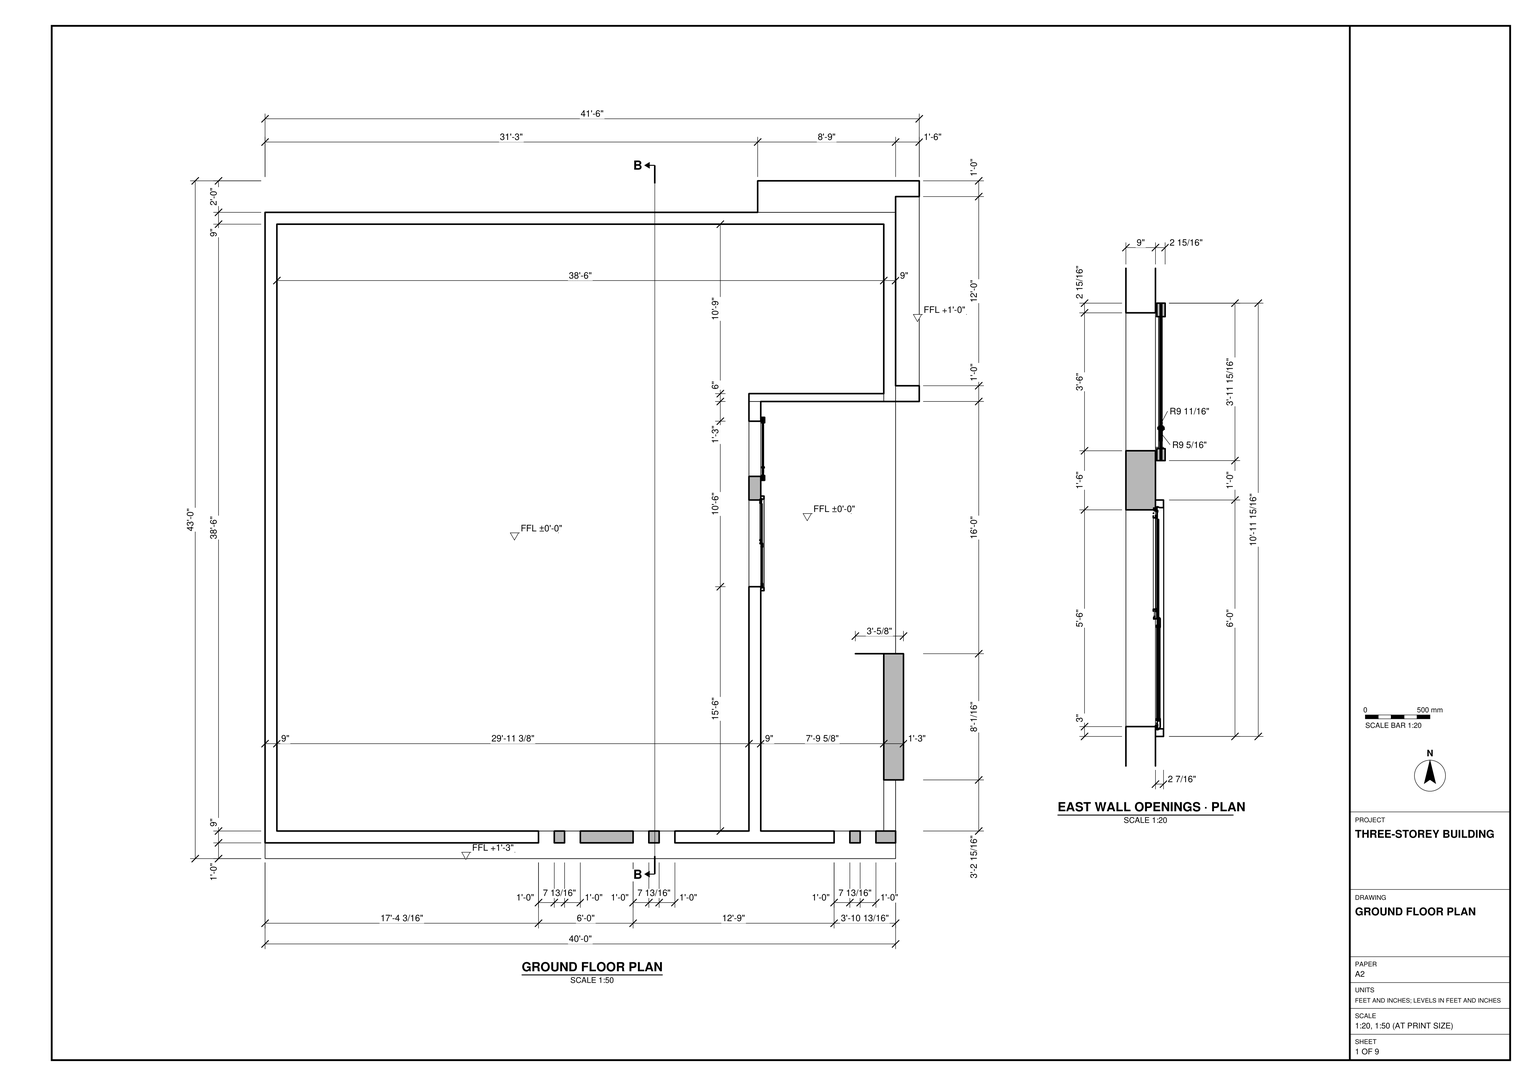
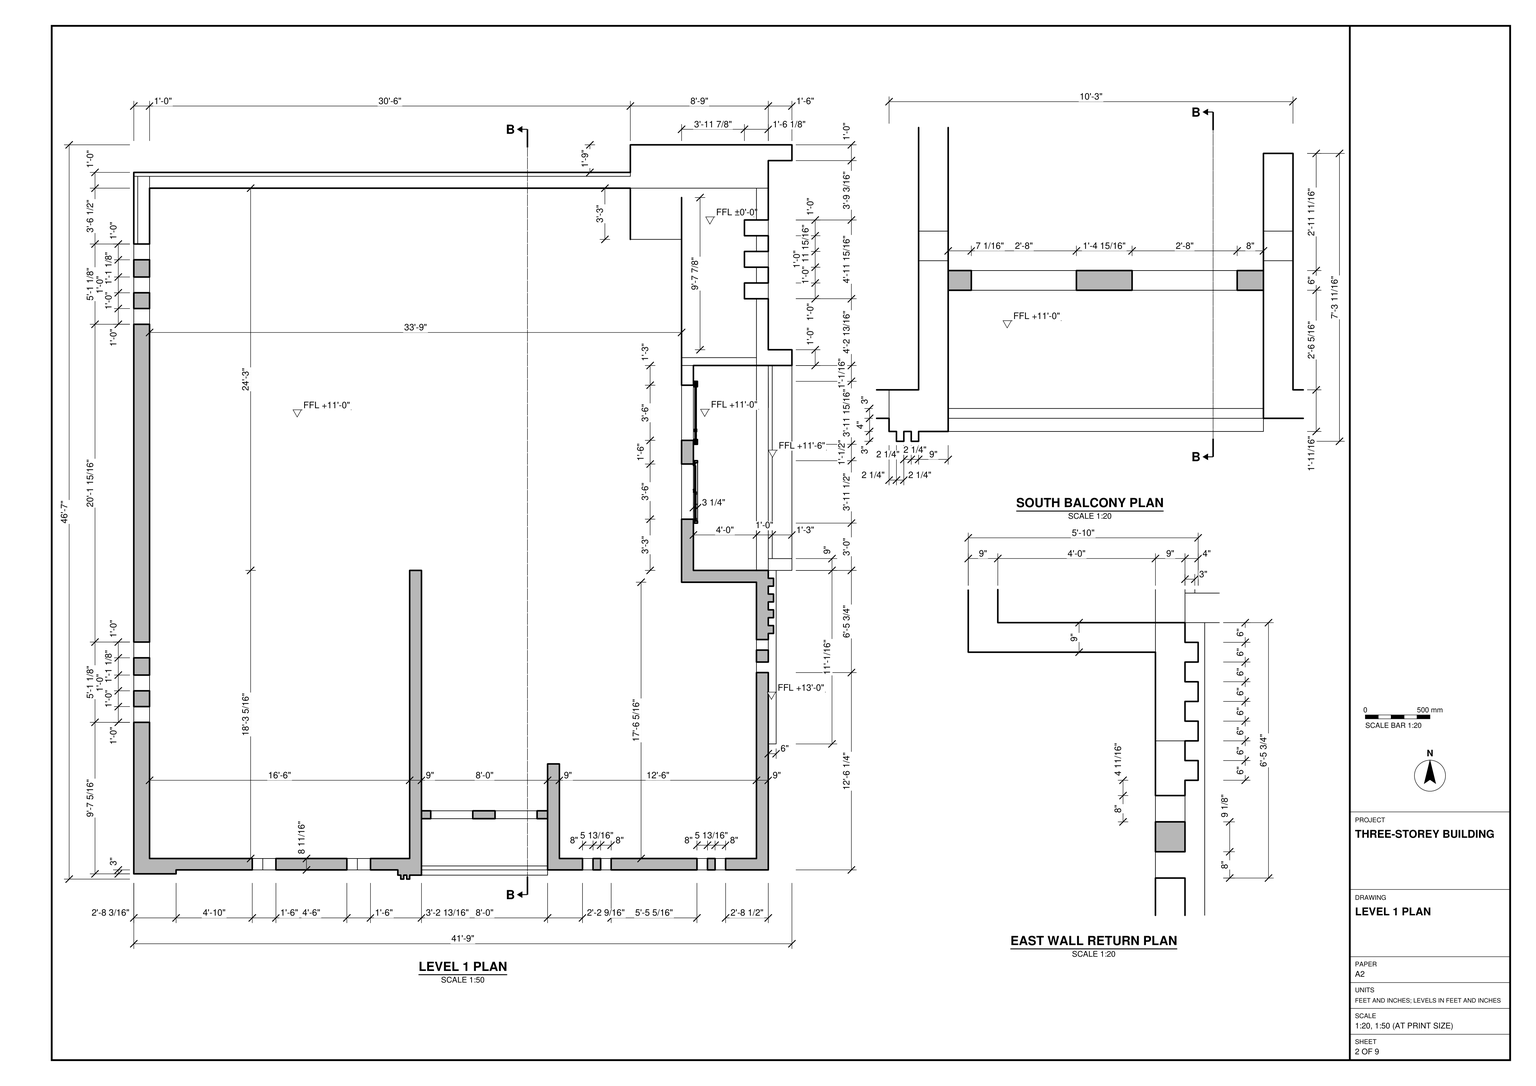
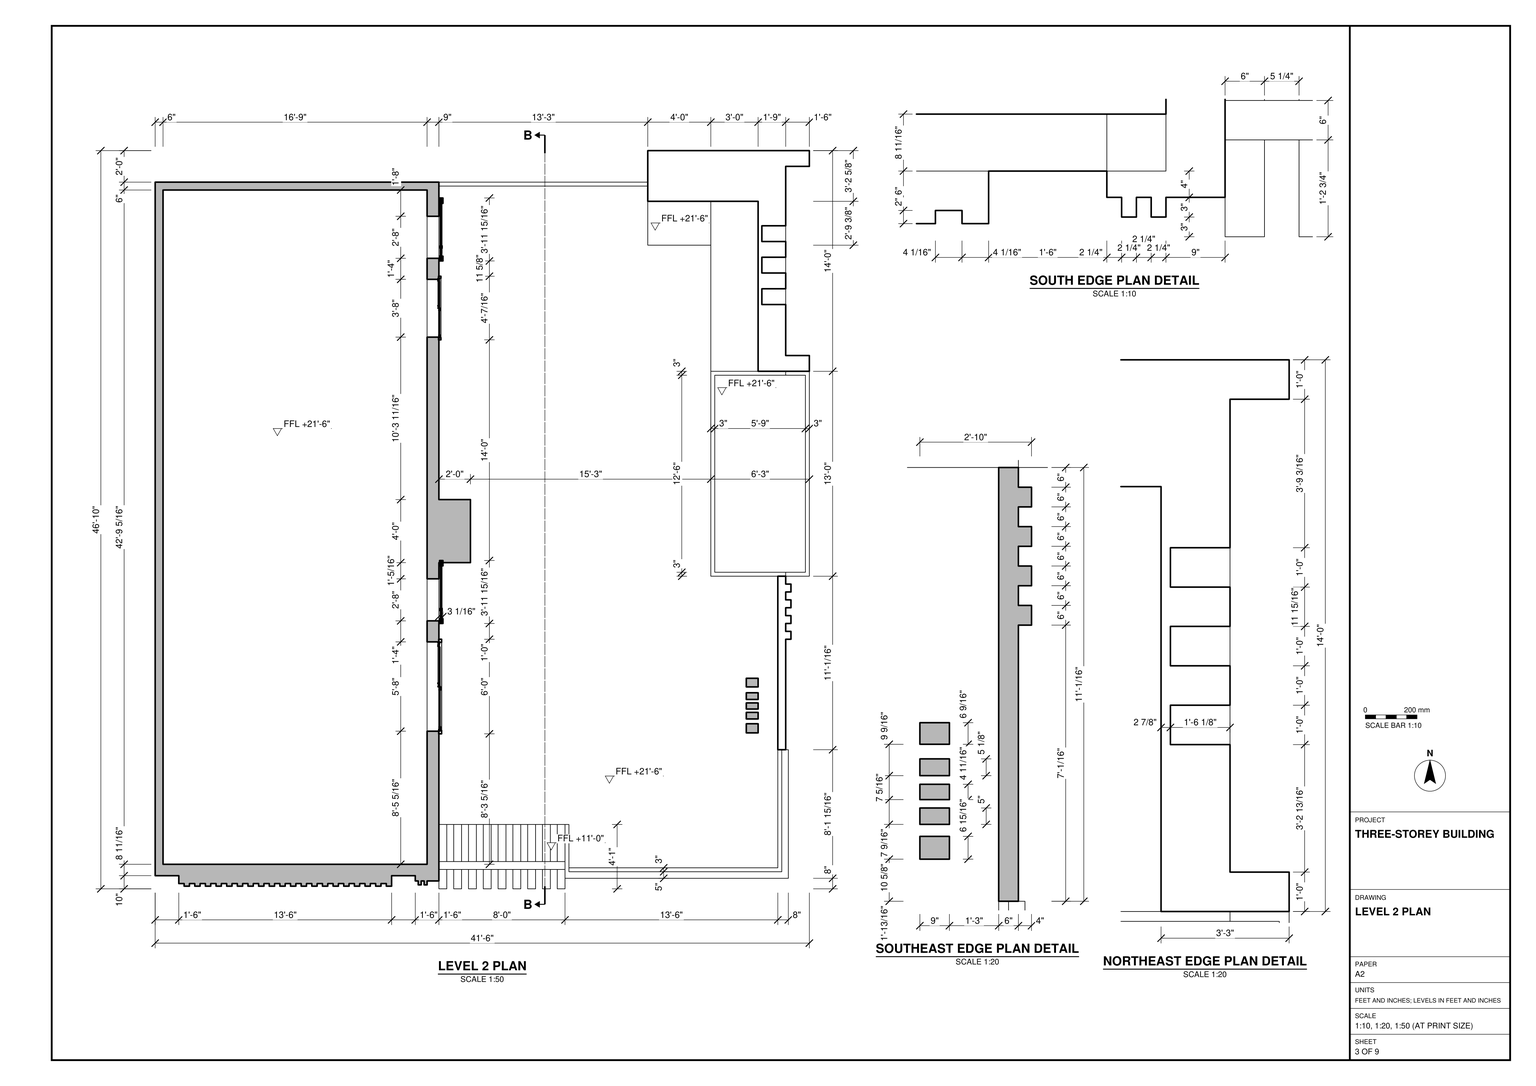
Build the three-storey building in SketchUp from task_files/diagram_01.pdf. Work in feet and inches. The overall model extents are 53'-5 5/16" along X, 49'-10 3/8" along Y and 37'-0" in height. Set the ground floor at ±0'-0", Level 1 at +11'-0" and Level 2 at +21'-6". Use the dimensioned wall lines on each plan, rather than the overall model extents, to lay out each floor.

On the ground floor, form the wide north end and the recessed east side. Use the east wall detail to place the openings and the pier between them. At Level 1, set the south balcony between the two projecting bays. Include the grouped west wall openings and the stepped return on the east side. At Level 2, distinguish the long enclosed space on the west from the open terrace on the east. Follow the enlarged details for the projections and recesses along the terrace edges.

Model the walls at their drawn thicknesses, with floor slabs, roof, door and window units, and balcony and terrace edges as shown. Include stairs, built-in joinery and main furniture where drawn. Keep shell elements such as walls, slabs and roof, and each furniture or joinery piece, in separate groups or components. Use components for repeated parts. Decor and loose items may be any suitable library components. Save one SketchUp model as output_files/three_storey_building_with_recessed_balcony_and_terrace.skp.

# SketchUp Ruby script. Lengths in inches.
U = 1.inch
M = Sketchup.active_model
def pt(a) = Geom::Point3d.new(a.map { |v| v * U })
def face(e, loops, mat)
  f = e.add_face(loops[0].map { |a| pt(a) })
  loops[1..].each { |l| e.add_face(l.map { |a| pt(a) }).erase! }
  f.material = f.back_material = mat if mat
  f
end
# faces: each face lists its corners as indices into pts; further lists are holes
def faces(e, pts, list, mat = nil) = list.each { |f| face(e, (f[0].is_a?(Array) ? f : [f]).map { |l| l.map { |i| pts[i] } }, mat) }
# xy, xz, yz: faces in a plane at the given z, y or x. An outline is a flat list of corners, or four numbers for a rectangle; further outlines are holes
def ring(l) = l.size == 4 ? [[l[0], l[1]], [l[2], l[1]], [l[2], l[3]], [l[0], l[3]]] : l.each_slice(2).to_a
def flat(e, list, mat, &to3) = list.each { |f| face(e, (f[0].is_a?(Array) ? f : [f]).map { |l| ring(l).map { |u, v| to3.(u, v) } }, mat) }
def xy(e, z, list, mat = nil) = flat(e, list, mat) { |x, y| [x, y, z] }
def xz(e, y, list, mat = nil) = flat(e, list, mat) { |x, z| [x, y, z] }
def yz(e, x, list, mat = nil) = flat(e, list, mat) { |y, z| [x, y, z] }
def lines(e, pts, list) = list.each { |a, b| e.add_line(pt(pts[a]), pt(pts[b])) }
# prism: a flat outline (further loops are holes) pulled along v
def prism(e, loops, v, mat = nil)
  f = face(e, loops, mat); d = Geom::Vector3d.new(v.map { |x| x * U })
  f.pushpull(f.normal.samedirection?(d) ? d.length : -d.length)
end
def box(e, o, s, mat = nil) = prism(e, [[o, [o[0] + s[0], o[1], o[2]], [o[0] + s[0], o[1] + s[1], o[2]], [o[0], o[1] + s[1], o[2]]]], [0, 0, s[2]], mat)
def at(x, y, z, deg = 0) = Geom::Transformation.translation(pt([x, y, z])) * Geom::Transformation.rotation(ORIGIN, Z_AXIS, deg.degrees)
def axes(o, x, y, z) = Geom::Transformation.new([*x, 0, *y, 0, *z, 0, *pt(o).to_a, 1])
def part(name) = M.definitions.add(name)
# library, detail: a bought-in or finely detailed component or shape, given as its bounding box
def library(name, o, s) = part(name).tap { |d| box(d.entities, o, s) }
def detail(e, o, s) = box(e.add_group.entities, o, s)
def put(e, d, t, mat = nil) = e.add_instance(d, t).tap { |i| i.material = mat if mat }
def group(e, t, mat = nil) = e.add_group.tap { |g| g.transformation = t; g.material = mat if mat }.entities
root = M.entities
M.materials.add("Brick_20_1K").color = [186, 180, 162]
M.materials.add("D01_Frost_White").color = [255, 242, 206]
M.materials.add("Glass_Basic_01").color = [161, 173, 186]
M.materials["Glass_Basic_01"].alpha = 0.25
M.materials.add("M05_Graphite_Haze").color = [114, 114, 114]
M.materials.add("M08_Obsidian_Black").color = [30, 30, 30]
M.materials.add("ThomThom - Waistcoat1").color = [155, 155, 155]
M.materials.add("Wood_Veneer_15_1K").color = [153, 101, 54]
M.materials.add("[Color_009]1").color = [0, 0, 0]
c1 = library("2016+Honda+Civic+LX+Sedan",[0.01,0.03,0.02],[16.17,34.46,10.62])
c2 = library("porta+4",[0.2,-5.42,1.33],[46.55,4.72,83.21])
c3 = library("mesh-165",[-1596.32,-2661.67,-39.91],[1702.88,1739.15,82.5])
c4 = part("Group15")
put(c4.entities,c3,at(294.66,859.51,3.5))
xy(root,288,[[240,556,399,559]])
xz(root,556,[[240,258,399,288]],"Glass_Basic_01")
xz(root,559,[[240,258,399,288]],"Glass_Basic_01")
p = [[504,451,96.6875],[504,571,96.6875]]
lines(root,p,[[0,1]])
put(root,c1,axes([537.55,376.82,0.04],[6.42482,0,0],[0,6.42482,0],[0,0,6.42482]))
g1 = group(root,at(33,88,0))
box(g1,[-9,-9,-6],[480,480,6])
g2 = group(root,at(24,79,0))
xy(g2,0,[[0,-12,0,480,375,480,375,504,498,504,498,336,471,336,471,471,9,471,9,9,368.36,9,368.36,336,377.36,336,377.36,9,471,9,471,144,486,144,486,47.91,480,47.91,480,-12],[368.36,336,471,342]])
xy(g2,7.84,[[368.36,279,377.36,321]])
xy(g2,12,[[480,348,498,492]],"M05_Graphite_Haze")
xy(g2,15,[[0,-12,480,-12,480,0,465.02,0,465.02,9,453.02,9,453.02,0,445.1875,0,445.1875,9,433.1875,9,433.1875,0,312,0,312,9,300,9,300,0,292.16,0,292.16,9,280.16,9,280.16,0,240,0,240,9,228,9,228,0,220.16,0,220.16,9,208.16,9,208.16,0,0,0],[471,9,480,47.91]])
xy(g2,43.84,[[368.36,195,377.36,261]])
xy(g2,51,[[68.23,0,76.23,9],[152.16,0,160.16,9]],"[Color_009]1")
xy(g2,75,[[423,336,453,342]],"Wood_Veneer_15_1K")
xy(g2,97.84,[[368.36,195,377.36,261],[368.36,279,377.36,321]])
xy(g2,99,[[68.23,0,76.23,9],[152.16,0,160.16,9]],"M05_Graphite_Haze")
xy(g2,105,[[423,336,453,342]],"Wood_Veneer_15_1K")
xy(g2,111,[[433.1875,0,445.1875,9],[453.02,0,465.02,9],[471,9,480,47.91]],"M05_Graphite_Haze")
xy(g2,111,[[208.16,0,220.16,9],[228,0,240,9],[280.16,0,292.16,9],[300,0,312,9]],"[Color_009]1")
xy(g2,114,[[200.25,-55,200.25,-52,198,-52,198,0,312,0,312,-52,207,-52,207,-55,204.75,-55,204.75,-52,202.5,-52,202.5,-55]],"[Color_009]1")
xy(g2,120,[[0,-48,198,0],[312,-48,480,0],[0,0,480,0,480,9,377.36,9,377.36,336,368.36,336,368.36,9,0,9],[0,9,9,480],[9,9,9,471,471,471,471,342,368.36,342,368.36,9],
  [368.36,336,471,342]])
xy(g2,120,[[471,144,486,180]],"Brick_20_1K")
xy(g2,120,[[377.36,9,377.36,336,498,336,498,180,471,180,471,9]],"Wood_Veneer_15_1K")
xy(g2,132,[[216,-45,312,-9],[9,-39.33,207,-39.33,207,180,216,180,216,-3,312,-3,312,32.67,321,32.67,321,-39.33,471,-39.33,471,171,414,171,414,432,375,432,375,471,9,471],[216,-9,312,-3],[423,180,471,336],[471,180,480,336],
  [480,180,480.43,180,480,336]])
xy(g2,134,[[272,-9,304,-3]])
xy(g2,135,[[414,279,423,321]])
xy(g2,138,[[480,189,480.4,189,480,336],[480.4,189,483,189,483,336,480,336],[483,189,498,336]])
xy(g2,139.39,[[-3,-51,0,480],[0,-51,29.1875,-48],[-3,480,375,483]],"Wood_Veneer_15_1K")
xy(g2,144,[[216,-52,312,-48],[216,-48,312,-45]])
xy(g2,145.98,[[338.59,-48,346.59,-39.33],[352.39,-48,360.39,-39.33],[425.71,-48,433.71,-39.33],[439.51,-48,447.51,-39.33]],"M08_Obsidian_Black")
xy(g2,150.99,[[-3,64.33,9,76.33],[-3,88.33,9,100.33],[-3,113.46,9,125.46],[-3,367.37,9,379.37],[-3,391.37,9,403.37],
  [-3,416.49,9,428.49]],"Wood_Veneer_15_1K")
xy(g2,156,[[480,47.91,486,47.91,486,180,480,180,480,174,484,174,484,168,480,168,480,162,484,162,484,156,480,156,480,150,484,150,484,144,480,144,480,138,484,138,484,132,480,132,480,110.23,471,110.23,471,102.23,480,102.23],[471,119.34,480,127.34]])
xy(g2,161.03,[[461.85,386.83,480,398.83],[461.85,410.83,480,422.83],[461.85,434.79,480,446.79]],"M05_Graphite_Haze")
xy(g2,168,[[480,180,498,189],[480,189,483,336]])
xy(g2,168,[[87.19,-48,95.19,-39.33],[95.19,-48,105.19,-39.33],[159.19,-48,167.19,-39.33],[167.19,-48,177.19,-39.33],[216,-48,312,-45]],"M08_Obsidian_Black")
xy(g2,170,[[223.05,-9,255.05,-3]])
xy(g2,171,[[414,219,423,261]])
xy(g2,202,[[223.05,-9,255.05,-3]])
xy(g2,213,[[414,219,423,261],[414,279,423,321]])
xy(g2,214,[[272,-9,304,-3]])
xy(g2,217.98,[[338.59,-48,346.59,-39.33],[352.39,-48,360.39,-39.33],[425.71,-48,433.71,-39.33],[439.51,-48,447.51,-39.33],[471,102.23,480,110.23],
  [471,119.34,480,127.34]],"M08_Obsidian_Black")
xy(g2,222.99,[[-3,64.33,9,76.33],[-3,88.33,9,100.33],[-3,113.46,9,125.46],[-3,367.37,9,379.37],[-3,391.37,9,403.37],
  [-3,416.49,9,428.49]],"Wood_Veneer_15_1K")
xy(g2,233.03,[[461.85,386.83,480,398.83],[461.85,410.83,480,422.83],[461.85,434.79,480,446.79]],"M05_Graphite_Haze")
xy(g2,240,[[87.19,-48,105.19,-39.33],[159.19,-48,177.19,-39.33]],"M08_Obsidian_Black")
xy(g2,240,[[-3,-51,29.1875,-51,29.1875,-48,0,-48,0,480,375,480,375,483,-3,483]],"Wood_Veneer_15_1K")
xy(g2,252,[[198,-48,198,-39.33,9,-39.33,9,471,312,471,312,-3,216,-3,216,180,207,180,207,-48],[321,-39.33,321,471,375,471,375,432,414,432,414,171,471,171,471,-39.33],[312,32.67,321,471],[414,171,471,171,471,180,423,180,423,432,414,432],[423,180,498,336]])
xy(g2,252,[[216,-52,222,-9],[227.26,-52,233.26,-9],[238.53,-52,244.53,-9],[249.79,-52,255.79,-9],[261.05,-52,267.05,-9],
  [272.3125,-52,278.3125,-9],[283.58,-52,289.58,-9],[294.84,-52,300.84,-9],[306.1,-52,312,-9]],"Wood_Veneer_15_1K")
xy(g2,258,[[198,-48,207,-39.33],[222,-43.25,227.26,-37.25],[227.26,-43.25,233.26,-37.25],[233.26,-43.25,238.53,-37.25],[238.53,-43.25,244.53,-37.25],
  [244.53,-43.25,249.79,-37.25],[249.79,-43.25,255.79,-37.25],[255.79,-43.25,261.05,-37.25],[261.05,-43.25,267.05,-37.25],[267.05,-43.25,272.3125,-37.25],
  [272.3125,-43.25,278.3125,-37.25],[278.3125,-43.25,283.58,-37.25],[283.58,-43.25,289.58,-37.25],[289.58,-43.25,294.84,-37.25],[294.84,-43.25,300.84,-37.25],
  [300.84,-43.25,306.1,-37.25],[306.1,-43.25,312,-37.25],[[315,-42,474,-42,474,180,423,180,423,432,375,432,375,480,216,480,216,238.34,240,238.34,240,190.34,216,190.34,216,-9,315,-9],[450,60.73,459,67.67],[450,95.72,459,102.29],[450,86.16,459,91.27],[450,71.32,459,76.32],[450,78.87,459,83.53]],[6,-39.33,207,474],[207,180,216,180,216,190.34,240,190.34,240,238.34,216,238.34,216,474,207,474],
  [423,180,480,180,480,183,426,183,426,333,480,333,480,336,423,336],[426,183,495,333],[423,336,459,465.39],[375,432,423,465.39]])
xy(g2,258,[[216,-58,222,-43.25],[227.26,-58,233.26,-43.25],[238.53,-58,244.53,-43.25],[249.79,-58,255.79,-43.25],[261.05,-58,267.05,-43.25],
  [272.3125,-58,278.3125,-43.25],[283.58,-58,289.58,-43.25],[294.84,-58,300.84,-43.25],[306.1,-58,312,-43.25],[216,-37.25,222,-9],
  [227.26,-37.25,233.26,-9],[238.53,-37.25,244.53,-9],[249.79,-37.25,255.79,-9],[261.05,-37.25,267.05,-9],[272.3125,-37.25,278.3125,-9],
  [283.58,-37.25,289.58,-9],[294.84,-37.25,300.84,-9],[306.1,-37.25,312,-9]],"Wood_Veneer_15_1K")
xy(g2,260,[[207,146,216,178],[207,422,216,454]])
xy(g2,264,[[216,-43.25,312,-37.25]],"Wood_Veneer_15_1K")
xy(g2,270,[[312,-48,480,-48,480,47.91,477,47.91,477,-45,315,-45,315,-9,312,-9],[315,-45,477,-45,477,47.91,474,47.91,474,-42,315,-42],[480,180,498,180,498,336,480,336,480,333,495,333,495,183,480,183]])
xy(g2,276,[[22.05,-56,22.05,-54,18,-54,18,-48,180,-48,180,-56,175.95,-56,175.95,-54,171.9,-54,171.9,-56,167.85,-56,167.85,-54,163.8,-54,163.8,-56,159.75,-56,159.75,-54,155.7,-54,155.7,-56,151.65,-56,151.65,-54,147.6,-54,147.6,-56,143.55,-56,143.55,-54,139.5,-54,139.5,-56,135.45,-56,135.45,-54,131.4,-54,131.4,-56,127.35,-56,127.35,-54,123.3,-54,123.3,-56,119.25,-56,119.25,-54,115.2,-54,115.2,-56,111.15,-56,111.15,-54,107.1,-54,107.1,-56,103.05,-56,103.05,-54,99,-54,99,-56,94.95,-56,94.95,-54,90.9,-54,90.9,-56,86.85,-56,86.85,-54,82.8,-54,82.8,-56,78.75,-56,78.75,-54,74.7,-54,74.7,-56,70.65,-56,70.65,-54,66.6,-54,66.6,-56,62.55,-56,62.55,-54,58.5,-54,58.5,-56,54.45,-56,54.45,-54,50.4,-54,50.4,-56,46.35,-56,46.35,-54,42.3,-54,42.3,-56,38.25,-56,38.25,-54,34.2,-54,34.2,-56,30.15,-56,30.15,-54,26.1,-54,26.1,-56]],"ThomThom - Waistcoat1")
xy(g2,287,[[312,-50,480,-48],[480,-50,482,47.91]],"Glass_Basic_01")
xy(g2,288,[[312,-50,482,-50,482,47.91,477,47.91,477,-45,315,-45,315,-9,312,-9]])
xy(g2,288,[[480,180,498,180,498,336,480,336,480,333,495,333,495,183,480,183]],"Glass_Basic_01")
xy(g2,290.04,[[461.85,386.83,480,398.83],[461.85,410.83,480,422.83],[461.85,434.79,480,446.79]],"M05_Graphite_Haze")
xy(g2,296,[[207,62,216,130],[207,362,216,406]])
xy(g2,312,[[474,47.91,480,47.91,480,132,484,132,484,138,480,138,480,144,484,144,484,150,480,150,480,156,484,156,484,162,480,162,480,168,484,168,484,174,480,174,480,180,474,180]])
xy(g2,340,[[207,62,216,130],[207,146,216,178],[207,362,216,406],[207,422,216,454]])
xy(g2,362.04,[[461.85,386.83,480,398.83],[461.85,410.83,480,422.83],[461.85,434.79,480,446.79]],"M05_Graphite_Haze")
xy(g2,366,[[22.05,-56,26.1,-56,26.1,-54,30.15,-54,30.15,-56,34.2,-56,34.2,-54,38.25,-54,38.25,-56,42.3,-56,42.3,-54,46.35,-54,46.35,-56,50.4,-56,50.4,-54,54.45,-54,54.45,-56,58.5,-56,58.5,-54,62.55,-54,62.55,-56,66.6,-56,66.6,-54,70.65,-54,70.65,-56,74.7,-56,74.7,-54,78.75,-54,78.75,-56,82.8,-56,82.8,-54,86.85,-54,86.85,-56,90.9,-56,90.9,-54,94.95,-54,94.95,-56,99,-56,99,-54,103.05,-54,103.05,-56,107.1,-56,107.1,-54,111.15,-54,111.15,-56,115.2,-56,115.2,-54,119.25,-54,119.25,-56,123.3,-56,123.3,-54,127.35,-54,127.35,-56,131.4,-56,131.4,-54,135.45,-54,135.45,-56,139.5,-56,139.5,-54,143.55,-54,143.55,-56,147.6,-56,147.6,-54,151.65,-54,151.65,-56,155.7,-56,155.7,-54,159.75,-54,159.75,-56,163.8,-56,163.8,-54,167.85,-54,167.85,-56,171.9,-56,171.9,-54,175.95,-54,175.95,-56,180,-56,180,-48,18,-48,18,-54,22.05,-54]],"ThomThom - Waistcoat1")
xy(g2,372,[[216,190.34,240,238.34]])
xy(g2,384,[[[-24,-79,312,504],[-18,-73,306,498]],[[-18,-73,306,498],[200.25,-55,202.5,-55,202.5,-52,204.75,-52,204.75,-55,207,-55,207,-52,216,-52,216,480,0,480,0,-48,198,-48,198,-52,200.25,-52]],[200.25,-55,200.25,-52,198,-52,198,-48,0,-48,0,-39.33,216,-39.33,216,-52,207,-52,207,-55,204.75,-55,204.75,-52,202.5,-52,202.5,-55],[0,-39.33,6,480],[6,-39.33,207,474],
  [207,-39.33,216,474],[6,474,216,480]])
xy(g2,390,[[-18,-73,306,498]])
xy(g2,390.94,[[312,5.5,312,26.83,417.58,26.83,417.58,48.15,312,48.15,312,102.29,417.35,102.29,417.35,112.125,312,112.125,312,133.45,417.58,133.45,417.58,154.78,312,154.78,312,176.1,417.58,176.1,417.58,197.43,312,197.43,312,218.75,417.35,218.75,417.35,240.08,312,240.08,312,261.4,417.35,261.4,417.35,282.73,312,282.73,312,304.05,417.35,304.05,417.35,325.375,312,325.375,312,346.7,417.35,346.7,417.35,368.03,312,368.03,312,389.35,417.35,389.35,417.35,410.68,312,410.68,312,432,450,432,450,5.5]])
xy(g2,409.59,[[312,5.5,366,26.83],[366,5.5,450,5.5,450,60.73,366,60.73,366,48.15,417.58,48.15,417.58,26.83,366,26.83],[312,48.15,366,60.73],[366,60.73,450,67.67],[312,67.67,366,69.48],
  [366,67.67,450,69.48],[312,69.48,366,71.32],[366,69.48,450,71.32],[366,71.32,450,76.32],[312,76.32,366,78.87],
  [366,76.32,450,78.87],[366,78.87,450,83.53],[312,83.53,366,86.16],[366,83.53,450,86.16],[366,86.16,450,90.8],
  [366,90.8,450,91.27],[312,91.27,366,95.72],[366,91.27,450,95.72],[366,95.72,450,102.29],[417.35,102.29,450,102.29,450,432,312,432,312,410.68,417.35,410.68,417.35,389.35,312,389.35,312,368.03,417.35,368.03,417.35,346.7,312,346.7,312,325.375,417.35,325.375,417.35,304.05,312,304.05,312,282.73,417.35,282.73,417.35,261.4,312,261.4,312,240.08,417.35,240.08,417.35,218.75,312,218.75,312,197.43,417.58,197.43,417.58,176.1,312,176.1,312,154.78,417.58,154.78,417.58,133.45,312,133.45,312,112.125,417.35,112.125]])
xy(g2,415.59,[[312,60.73,459,67.67],[312,71.32,459,76.32],[312,78.87,459,83.53],[312,86.16,459,91.27],[312,95.72,459,102.29]])
xy(g2,426,[[-24,-79,312,-79,312,465.39,306,465.39,306,-73,-18,-73,-18,465.39,-24,465.39],[-24,465.39,-18,504],[-18,465.39,306,498],[306,465.39,312,504],[312,465.39,375,504],
  [-18,498,306,504]])
xy(g2,426,[[480,348,498,492]],"M05_Graphite_Haze")
xy(g2,438,[[459,336,498,336,498,504,-24,504,-24,465.39,459,465.39]])
xz(g2,-79,[[-24,384,312,426]])
xz(g2,-73,[[-18,390,306,426]])
xz(g2,-58,[[216,255,222,258],[227.26,255,233.26,258],[238.53,255,244.53,258],[249.79,255,255.79,258],[261.05,255,267.05,258],
  [272.3125,255,278.3125,258],[283.58,255,289.58,258],[294.84,255,300.84,258],[306.1,255,312,258]],"Wood_Veneer_15_1K")
xz(g2,-56,[[22.05,276,26.1,366],[30.15,276,34.2,366],[38.25,276,42.3,366],[46.35,276,50.4,366],[54.45,276,58.5,366],
  [62.55,276,66.6,366],[70.65,276,74.7,366],[78.75,276,82.8,366],[86.85,276,90.9,366],[94.95,276,99,366],
  [103.05,276,107.1,366],[111.15,276,115.2,366],[119.25,276,123.3,366],[127.35,276,131.4,366],[135.45,276,139.5,366],
  [143.55,276,147.6,366],[151.65,276,155.7,366],[159.75,276,163.8,366],[167.85,276,171.9,366],[175.95,276,180,366]],"ThomThom - Waistcoat1")
xz(g2,-55,[[200.25,114,202.5,384],[204.75,114,207,384]])
xz(g2,-54,[[18,276,22.05,366],[26.1,276,30.15,366],[34.2,276,38.25,366],[42.3,276,46.35,366],[50.4,276,54.45,366],
  [58.5,276,62.55,366],[66.6,276,70.65,366],[74.7,276,78.75,366],[82.8,276,86.85,366],[90.9,276,94.95,366],
  [99,276,103.05,366],[107.1,276,111.15,366],[115.2,276,119.25,366],[123.3,276,127.35,366],[131.4,276,135.45,366],
  [139.5,276,143.55,366],[147.6,276,151.65,366],[155.7,276,159.75,366],[163.8,276,167.85,366],[171.9,276,175.95,366]],"ThomThom - Waistcoat1")
xz(g2,-52,[[198,114,200.25,384],[202.5,114,204.75,384]])
xz(g2,-52,[[207,114,312,114,312,144,216,144,216,384,207,384]],"M05_Graphite_Haze")
xz(g2,-51,[[-3,139.39,29.1875,240]],"Wood_Veneer_15_1K")
xz(g2,-50,[[312,287,482,288]],"M08_Obsidian_Black")
xz(g2,-48,[[[0,120,198,120,198,384,0,384,0,240,29.1875,240,29.1875,139.39,0,139.39],[18,276,180,366],[159.19,168,177.19,240],[87.19,168,105.19,240]],[312,120,480,132],[312,246,480,270],[198,252,207,258]])
xz(g2,-48,[[216,144,312,168],[312,270,480,287]],"Glass_Basic_01")
xz(g2,-48,[[[312,132,480,246],[439.51,145.98,447.51,217.98],[338.59,145.98,346.59,217.98],[352.39,145.98,360.39,217.98],[425.71,145.98,433.71,217.98]]],"Wood_Veneer_15_1K")
xz(g2,-45,[[216,132,312,144],[216,144,312,168],[315,270,477,288]],"Glass_Basic_01")
xz(g2,-43.25,[[216,258,312,264]],"Wood_Veneer_15_1K")
xz(g2,-42,[[315,258,474,270]])
xz(g2,-39.33,[[[9,132,9,252,198,252,198,258,207,258,207,132],[87.19,168,105.19,240],[159.19,168,177.19,240]],[[321,132,471,252],[352.39,145.98,360.39,217.98],[338.59,145.98,346.59,217.98],[439.51,145.98,447.51,217.98],[425.71,145.98,433.71,217.98]],[6,258,207,384]])
xz(g2,-37.25,[[216,258,312,264]],"Wood_Veneer_15_1K")
xz(g2,-12,[[0,0,480,15]])
xz(g2,-9,[[[216,132,270,132,270,216,306,216,306,132,312,132,312,252,306.1,252,306.1,258,300.84,258,300.84,252,294.84,252,294.84,258,289.58,258,289.58,252,283.58,252,283.58,258,278.3125,258,278.3125,252,272.3125,252,272.3125,258,267.05,258,267.05,252,261.05,252,261.05,258,255.79,258,255.79,252,249.79,252,249.79,258,244.53,258,244.53,252,238.53,252,238.53,258,233.26,258,233.26,252,227.26,252,227.26,258,222,258,222,252,216,252],[221.05,168,257.05,204]],[[270,132,306,216],[272,134,304,214]],[[221.05,168,257.05,204],[223.05,170,255.05,202]],[227.26,252,233.26,258],[238.53,252,244.53,258],
  [249.79,252,255.79,258],[261.05,252,267.05,258],[272.3125,252,278.3125,258],[283.58,252,289.58,258],[294.84,252,300.84,258],
  [306.1,252,312,258],[312,252,312.1,258],[312,258,315,270],[312,270,315,288]])
xz(g2,-3,[[[216,132,312,252],[272,134,304,214],[223.05,170,255.05,202]]])
xz(g2,0,[[198,114,312,120]])
xz(g2,0,[[[0,15,208.16,15,208.16,111,220.16,111,220.16,15,228,15,228,111,240,111,240,15,280.16,15,280.16,111,292.16,111,292.16,15,300,15,300,111,312,111,312,114,198,114,198,120,0,120],[152.16,51,160.16,99],[68.23,51,76.23,99]],[312,15,433.1875,15,433.1875,111,445.1875,111,445.1875,15,453.02,15,453.02,111,465.02,111,465.02,15,480,15,480,120,312,120]],"M05_Graphite_Haze")
xz(g2,5.5,[[312,390.94,450,409.59]])
xz(g2,9,[[[9,0,368.36,120],[280.16,15,292.16,111],[300,15,312,111],[228,15,240,111],[208.16,15,220.16,111],[152.16,51,160.16,99],[68.23,51,76.23,99]],[[377.36,0,471,120],[453.02,15,465.02,111],[433.1875,15,445.1875,111]]])
xz(g2,9,[[471,15,480,111]],"M05_Graphite_Haze")
xz(g2,26.83,[[312,390.94,417.58,409.59]])
xz(g2,32.67,[[312,132,321,252]])
xz(g2,47.91,[[474,270,477,270,477,288,480,288,480,312,474,312],[477,270,480,288]])
xz(g2,47.91,[[480,0,486,156]],"Brick_20_1K")
xz(g2,47.91,[[471,15,480,111]],"M05_Graphite_Haze")
xz(g2,47.91,[[480,287,482,288]],"M08_Obsidian_Black")
xz(g2,48.15,[[312,390.94,417.58,409.59]])
xz(g2,60.73,[[450,258,459,258,459,415.59,312,415.59,312,409.59,450,409.59]])
xz(g2,62,[[207,296,216,340]])
xz(g2,64.33,[[-3,150.99,9,222.99]],"Wood_Veneer_15_1K")
xz(g2,67.67,[[450,258,450,409.59,312,409.59,312,415.59,459,415.59,459,258]])
xz(g2,71.32,[[450,258,459,258,459,415.59,312,415.59,312,409.59,450,409.59]])
xz(g2,76.32,[[450,258,450,409.59,312,409.59,312,415.59,459,415.59,459,258]])
xz(g2,76.33,[[-3,150.99,9,222.99]],"Wood_Veneer_15_1K")
xz(g2,78.87,[[450,258,459,258,459,415.59,312,415.59,312,409.59,450,409.59]])
xz(g2,83.53,[[450,258,450,409.59,312,409.59,312,415.59,459,415.59,459,258]])
xz(g2,86.16,[[450,258,459,258,459,415.59,312,415.59,312,409.59,450,409.59]])
xz(g2,88.33,[[-3,150.99,9,222.99]],"Wood_Veneer_15_1K")
xz(g2,91.27,[[450,258,450,409.59,312,409.59,312,415.59,459,415.59,459,258]])
xz(g2,95.72,[[450,258,459,258,459,415.59,312,415.59,312,409.59,450,409.59]])
xz(g2,100.33,[[-3,150.99,9,222.99]],"Wood_Veneer_15_1K")
xz(g2,102.23,[[471,156,480,217.98]],"M08_Obsidian_Black")
xz(g2,102.29,[[450,258,450,409.59,417.35,409.59,417.35,390.94,312,390.94,312,415.59,459,415.59,459,258]])
xz(g2,110.23,[[471,156,480,217.98]],"M08_Obsidian_Black")
xz(g2,112.125,[[312,390.94,417.35,409.59]])
xz(g2,113.46,[[-3,150.99,9,222.99]],"Wood_Veneer_15_1K")
xz(g2,119.34,[[471,156,480,217.98]],"M08_Obsidian_Black")
xz(g2,125.46,[[-3,150.99,9,222.99]],"Wood_Veneer_15_1K")
xz(g2,127.34,[[471,156,480,217.98]],"M08_Obsidian_Black")
xz(g2,130,[[207,296,216,340]])
xz(g2,132,[[480,156,484,312]])
xz(g2,133.45,[[312,390.94,417.58,409.59]])
xz(g2,138,[[480,156,484,312]])
xz(g2,144,[[449.36,0,471,120],[480,156,484,312]])
xz(g2,144,[[471,0,486,120]],"Brick_20_1K")
xz(g2,146,[[207,260,216,340]])
xz(g2,150,[[480,156,484,312]])
xz(g2,154.78,[[312,390.94,417.58,409.59]])
xz(g2,156,[[480,156,484,312]])
xz(g2,162,[[480,156,484,312]])
xz(g2,168,[[480,156,484,312]])
xz(g2,171,[[414,132,471,252]])
xz(g2,174,[[480,156,484,312]])
xz(g2,176.1,[[312,390.94,417.58,409.59]])
xz(g2,178,[[207,260,216,340]])
xz(g2,180,[[207,132,216,252],[423,132,471,252],[471,132,480,252],[480,132,486,156],[207,252,216,258],
  [471,252,480,258],[480,252,498,270],[474,258,480,312]])
xz(g2,180,[[480,270,498,287]],"Glass_Basic_01")
xz(g2,180,[[486,120,498,120,498,168,480,168,480,156,486,156]],"M05_Graphite_Haze")
xz(g2,180,[[480,287,498,288]],"M08_Obsidian_Black")
xz(g2,183,[[480,258,495,270]])
xz(g2,183,[[480,270,495,288]],"Glass_Basic_01")
xz(g2,189,[[480,138,483,168],[483,138,498,168]])
xz(g2,190.34,[[216,258,240,372]],"M05_Graphite_Haze")
xz(g2,195,[[368.36,43.84,377.36,97.84]])
xz(g2,197.43,[[312,390.94,417.58,409.59]])
xz(g2,218.75,[[312,390.94,417.35,409.59]])
xz(g2,219,[[414,171,423,213]])
xz(g2,238.34,[[216,258,240,372]],"M05_Graphite_Haze")
xz(g2,240.08,[[312,390.94,417.35,409.59]])
xz(g2,261,[[368.36,43.84,377.36,97.84],[414,171,423,213]])
xz(g2,261.4,[[312,390.94,417.35,409.59]])
xz(g2,279,[[368.36,7.84,377.36,97.84],[414,135,423,213]])
xz(g2,282.73,[[312,390.94,417.35,409.59]])
xz(g2,304.05,[[312,390.94,417.35,409.59]])
xz(g2,321,[[368.36,7.84,377.36,97.84],[414,135,423,213]])
xz(g2,325.375,[[312,390.94,417.35,409.59]])
xz(g2,333,[[480,258,495,270]])
xz(g2,333,[[480,270,495,288]],"Glass_Basic_01")
xz(g2,336,[[480,138,483,168],[423,252,498,258],[480,258,498,270]])
xz(g2,336,[[480,270,498,287]],"Glass_Basic_01")
xz(g2,336,[[423,132,480,132,480,168,498,168,498,252,423,252],[480,132,498,138],[483,138,498,168],[459,258,480,258,480,288,498,288,498,438,459,438]],"M05_Graphite_Haze")
xz(g2,336,[[480,287,498,288]],"M08_Obsidian_Black")
xz(g2,336,[[[377.36,0,498,120],[420,72,456,108]],[[420,72,456,108],[423,75,453,105]]],"Wood_Veneer_15_1K")
xz(g2,342,[[[368.36,0,471,120],[423,75,453,105]]])
xz(g2,346.7,[[312,390.94,417.35,409.59]])
xz(g2,348,[[480,12,498,426]],"M05_Graphite_Haze")
xz(g2,362,[[207,296,216,340]])
xz(g2,367.37,[[-3,150.99,9,222.99]],"Wood_Veneer_15_1K")
xz(g2,368.03,[[312,390.94,417.35,409.59]])
xz(g2,379.37,[[-3,150.99,9,222.99]],"Wood_Veneer_15_1K")
xz(g2,386.83,[[461.85,161.03,480,233.03],[461.85,290.04,480,362.04]],"M05_Graphite_Haze")
xz(g2,389.35,[[312,390.94,417.35,409.59]])
xz(g2,391.37,[[-3,150.99,9,222.99]],"Wood_Veneer_15_1K")
xz(g2,398.83,[[461.85,161.03,480,233.03],[461.85,290.04,480,362.04]],"M05_Graphite_Haze")
xz(g2,403.37,[[-3,150.99,9,222.99]],"Wood_Veneer_15_1K")
xz(g2,406,[[207,296,216,340]])
xz(g2,410.68,[[312,390.94,417.35,409.59]])
xz(g2,410.83,[[461.85,161.03,480,233.03],[461.85,290.04,480,362.04]],"M05_Graphite_Haze")
xz(g2,416.49,[[-3,150.99,9,222.99]],"Wood_Veneer_15_1K")
xz(g2,422,[[207,260,216,340]])
xz(g2,422.83,[[461.85,161.03,480,233.03],[461.85,290.04,480,362.04]],"M05_Graphite_Haze")
xz(g2,428.49,[[-3,150.99,9,222.99]],"Wood_Veneer_15_1K")
xz(g2,432,[[375,252,423,258],[312,390.94,450,409.59]])
xz(g2,434.79,[[461.85,161.03,480,233.03],[461.85,290.04,480,362.04]],"M05_Graphite_Haze")
xz(g2,446.79,[[461.85,161.03,480,233.03],[461.85,290.04,480,362.04]],"M05_Graphite_Haze")
xz(g2,454,[[207,260,216,340]])
xz(g2,465.39,[[375,258,459,258,459,438,-24,438,-24,426,375,426]])
xz(g2,471,[[9,0,471,120],[9,132,375,252]])
xz(g2,474,[[6,258,207,384]])
xz(g2,480,[[0,0,375,120],[0,120,375,139.39],[0,240,375,258],[0,258,216,384]])
xz(g2,483,[[-3,139.39,375,240]],"Wood_Veneer_15_1K")
xz(g2,492,[[480,12,498,426]],"M05_Graphite_Haze")
xz(g2,498,[[-18,390,306,426]])
xz(g2,504,[[375,0,375,426,-24,426,-24,438,498,438,498,0],[-24,384,312,426]])
yz(g2,-24,[[-79,384,504,426],[465.39,426,504,438]])
yz(g2,-18,[[-73,390,498,426]])
yz(g2,-3,[[[-51,139.39,483,240],[64.33,150.99,76.33,222.99],[88.33,150.99,100.33,222.99],[113.46,150.99,125.46,222.99],[367.37,150.99,379.37,222.99],[391.37,150.99,403.37,222.99],[416.49,150.99,428.49,222.99]]],"Wood_Veneer_15_1K")
yz(g2,0,[[-12,0,-12,15,0,15,0,120,480,120,480,0],[-48,120,480,139.39],[-48,240,480,258],[-48,258,480,384]])
yz(g2,6,[[-39.33,258,474,384]])
yz(g2,9,[[9,0,471,120],[[-39.33,132,471,252],[367.37,150.99,379.37,222.99],[391.37,150.99,403.37,222.99],[416.49,150.99,428.49,222.99],[113.46,150.99,125.46,222.99],[88.33,150.99,100.33,222.99],[64.33,150.99,76.33,222.99]]])
yz(g2,18,[[-54,276,-48,366]],"ThomThom - Waistcoat1")
yz(g2,22.05,[[-56,276,-54,366]],"ThomThom - Waistcoat1")
yz(g2,26.1,[[-56,276,-54,366]],"ThomThom - Waistcoat1")
yz(g2,29.1875,[[-51,139.39,-48,240]],"Wood_Veneer_15_1K")
yz(g2,30.15,[[-56,276,-54,366]],"ThomThom - Waistcoat1")
yz(g2,34.2,[[-56,276,-54,366]],"ThomThom - Waistcoat1")
yz(g2,38.25,[[-56,276,-54,366]],"ThomThom - Waistcoat1")
yz(g2,42.3,[[-56,276,-54,366]],"ThomThom - Waistcoat1")
yz(g2,46.35,[[-56,276,-54,366]],"ThomThom - Waistcoat1")
yz(g2,50.4,[[-56,276,-54,366]],"ThomThom - Waistcoat1")
yz(g2,54.45,[[-56,276,-54,366]],"ThomThom - Waistcoat1")
yz(g2,58.5,[[-56,276,-54,366]],"ThomThom - Waistcoat1")
yz(g2,62.55,[[-56,276,-54,366]],"ThomThom - Waistcoat1")
yz(g2,66.6,[[-56,276,-54,366]],"ThomThom - Waistcoat1")
yz(g2,68.23,[[0,51,9,99]],"[Color_009]1")
yz(g2,70.65,[[-56,276,-54,366]],"ThomThom - Waistcoat1")
yz(g2,74.7,[[-56,276,-54,366]],"ThomThom - Waistcoat1")
yz(g2,76.23,[[0,51,9,99]],"[Color_009]1")
yz(g2,78.75,[[-56,276,-54,366]],"ThomThom - Waistcoat1")
yz(g2,82.8,[[-56,276,-54,366]],"ThomThom - Waistcoat1")
yz(g2,86.85,[[-56,276,-54,366]],"ThomThom - Waistcoat1")
yz(g2,87.19,[[-48,168,-39.33,240]],"M08_Obsidian_Black")
yz(g2,90.9,[[-56,276,-54,366]],"ThomThom - Waistcoat1")
yz(g2,94.95,[[-56,276,-54,366]],"ThomThom - Waistcoat1")
yz(g2,99,[[-56,276,-54,366]],"ThomThom - Waistcoat1")
yz(g2,103.05,[[-56,276,-54,366]],"ThomThom - Waistcoat1")
yz(g2,105.19,[[-48,168,-39.33,240]],"M08_Obsidian_Black")
yz(g2,107.1,[[-56,276,-54,366]],"ThomThom - Waistcoat1")
yz(g2,111.15,[[-56,276,-54,366]],"ThomThom - Waistcoat1")
yz(g2,115.2,[[-56,276,-54,366]],"ThomThom - Waistcoat1")
yz(g2,119.25,[[-56,276,-54,366]],"ThomThom - Waistcoat1")
yz(g2,123.3,[[-56,276,-54,366]],"ThomThom - Waistcoat1")
yz(g2,127.35,[[-56,276,-54,366]],"ThomThom - Waistcoat1")
yz(g2,131.4,[[-56,276,-54,366]],"ThomThom - Waistcoat1")
yz(g2,135.45,[[-56,276,-54,366]],"ThomThom - Waistcoat1")
yz(g2,139.5,[[-56,276,-54,366]],"ThomThom - Waistcoat1")
yz(g2,143.55,[[-56,276,-54,366]],"ThomThom - Waistcoat1")
yz(g2,147.6,[[-56,276,-54,366]],"ThomThom - Waistcoat1")
yz(g2,151.65,[[-56,276,-54,366]],"ThomThom - Waistcoat1")
yz(g2,152.16,[[0,51,9,99]],"[Color_009]1")
yz(g2,155.7,[[-56,276,-54,366]],"ThomThom - Waistcoat1")
yz(g2,159.19,[[-48,168,-39.33,240]],"M08_Obsidian_Black")
yz(g2,159.75,[[-56,276,-54,366]],"ThomThom - Waistcoat1")
yz(g2,160.16,[[0,51,9,99]],"[Color_009]1")
yz(g2,163.8,[[-56,276,-54,366]],"ThomThom - Waistcoat1")
yz(g2,167.85,[[-56,276,-54,366]],"ThomThom - Waistcoat1")
yz(g2,171.9,[[-56,276,-54,366]],"ThomThom - Waistcoat1")
yz(g2,175.95,[[-56,276,-54,366]],"ThomThom - Waistcoat1")
yz(g2,177.19,[[-48,168,-39.33,240]],"M08_Obsidian_Black")
yz(g2,180,[[-56,276,-48,366]],"ThomThom - Waistcoat1")
yz(g2,198,[[-52,114,-48,132],[-48,114,0,120],[-52,132,-48,384],[-48,252,-39.33,258]])
yz(g2,200.25,[[-55,114,-52,384]])
yz(g2,202.5,[[-55,114,-52,384]])
yz(g2,204.75,[[-55,114,-52,384]])
yz(g2,207,[[-55,114,-52,384],[-39.33,132,180,252],[-48,252,-39.33,258],[-39.33,252,180,258],[[-39.33,258,474,384],[62,296,130,340],[422,260,454,340],[146,260,178,340],[362,296,406,340]]])
yz(g2,208.16,[[0,15,9,111]],"[Color_009]1")
yz(g2,216,[[-9,132,-3,132,-3,252,180,252,180,258,-37.25,258,-37.25,264,-43.25,264,-43.25,258,-52,258,-52,252,-9,252],[-3,132,180,252],[-48,144,-45,168],[[-9,258,144,258,144,342,180,342,180,258,190.34,258,190.34,372,-9,372],[60,294,132,342]],[[144,258,180,342],[146,260,178,340]],
  [[238.34,258,420,258,420,342,456,342,456,258,468,258,468,372,238.34,372],[360,294,408,342]],[[420,258,456,342],[422,260,454,340]],[[60,294,132,342],[62,296,130,340]],[[360,294,408,342],[362,296,406,340]]])
yz(g2,216,[[-45,132,-9,132,-9,252,-52,252,-52,144,-48,144,-48,168,-45,168],[-52,258,-43.25,258,-43.25,264,-37.25,264,-37.25,258,-9,258,-9,372,468,372,468,258,480,258,480,384,-52,384]],"M05_Graphite_Haze")
yz(g2,216,[[-52,252,-58,255,-52,255],[-58,255,-52,258]],"Wood_Veneer_15_1K")
yz(g2,220.16,[[0,15,9,111]],"[Color_009]1")
yz(g2,222,[[-52,252,-9,252,-9,258,-58,258,-58,255]],"Wood_Veneer_15_1K")
yz(g2,223.05,[[-9,170,-3,202]])
yz(g2,227.26,[[-52,252,-58,255,-58,258,-9,258,-9,252]],"Wood_Veneer_15_1K")
yz(g2,228,[[0,15,9,111]],"[Color_009]1")
yz(g2,233.26,[[-52,252,-9,252,-9,258,-58,258,-58,255]],"Wood_Veneer_15_1K")
yz(g2,238.53,[[-52,252,-58,255,-58,258,-9,258,-9,252]],"Wood_Veneer_15_1K")
yz(g2,240,[[190.34,258,238.34,372]],"M05_Graphite_Haze")
yz(g2,240,[[0,15,9,111]],"[Color_009]1")
yz(g2,244.53,[[-52,252,-9,252,-9,258,-58,258,-58,255]],"Wood_Veneer_15_1K")
yz(g2,249.79,[[-52,252,-58,255,-58,258,-9,258,-9,252]],"Wood_Veneer_15_1K")
yz(g2,255.05,[[-9,170,-3,202]])
yz(g2,255.79,[[-52,252,-9,252,-9,258,-58,258,-58,255]],"Wood_Veneer_15_1K")
yz(g2,261.05,[[-52,252,-58,255,-58,258,-9,258,-9,252]],"Wood_Veneer_15_1K")
yz(g2,267.05,[[-52,252,-9,252,-9,258,-58,258,-58,255]],"Wood_Veneer_15_1K")
yz(g2,272,[[-9,134,-3,214]])
yz(g2,272.3125,[[-52,252,-58,255,-58,258,-9,258,-9,252]],"Wood_Veneer_15_1K")
yz(g2,278.3125,[[-52,252,-9,252,-9,258,-58,258,-58,255]],"Wood_Veneer_15_1K")
yz(g2,280.16,[[0,15,9,111]],"[Color_009]1")
yz(g2,283.58,[[-52,252,-58,255,-58,258,-9,258,-9,252]],"Wood_Veneer_15_1K")
yz(g2,289.58,[[-52,252,-9,252,-9,258,-58,258,-58,255]],"Wood_Veneer_15_1K")
yz(g2,292.16,[[0,15,9,111]],"[Color_009]1")
yz(g2,294.84,[[-52,252,-58,255,-58,258,-9,258,-9,252]],"Wood_Veneer_15_1K")
yz(g2,300,[[0,15,9,111]],"[Color_009]1")
yz(g2,300.84,[[-52,252,-9,252,-9,258,-58,258,-58,255]],"Wood_Veneer_15_1K")
yz(g2,304,[[-9,134,-3,214]])
yz(g2,306,[[-73,390,498,426]])
yz(g2,306.1,[[-52,252,-58,255,-58,258,-9,258,-9,252]],"Wood_Veneer_15_1K")
yz(g2,312,[[-52,114,0,114,0,120,-48,120,-48,144,-52,144],[-45,132,-45,168,-48,168,-48,252,-9,252,-9,132],[-48,132,-45,144],[-9,132,-3,252],[-3,132,32.67,252],
  [-48,144,-45,168],[-48,252,-9,258],[-48,258,-48,270,-9,270,-9,264,-43.25,264,-43.25,258],[-37.25,258,-9,264],[[-79,384,504,426],[48.15,390.94,48.15,409.59,60.73,409.59,60.73,415.59,67.67,415.59,67.67,409.59,71.32,409.59,71.32,415.59,76.32,415.59,76.32,409.59,78.87,409.59,78.87,415.59,83.53,415.59,83.53,409.59,86.16,409.59,86.16,415.59,91.27,415.59,91.27,409.59,95.72,409.59,95.72,415.59,102.29,415.59,102.29,390.94],[410.68,390.94,432,409.59],[5.5,390.94,26.83,409.59],[368.03,390.94,389.35,409.59],[282.73,390.94,304.05,409.59],[325.375,390.94,346.7,409.59],[240.08,390.94,261.4,409.59],[197.43,390.94,218.75,409.59],[154.78,390.94,176.1,409.59],[112.125,390.94,133.45,409.59]]])
yz(g2,312,[[-48,270,-48,287,-50,287,-50,288,-9,288,-9,270]],"Glass_Basic_01")
yz(g2,312,[[-52,252,-48,252,-48,258,-58,258,-58,255],[-43.25,258,-37.25,264]],"Wood_Veneer_15_1K")
yz(g2,312,[[0,15,9,111]],"[Color_009]1")
yz(g2,315,[[-42,258,-9,264],[-42,264,-9,270]])
yz(g2,315,[[-45,270,-9,288]],"Glass_Basic_01")
yz(g2,321,[[-39.33,132,32.67,252]])
yz(g2,338.59,[[-48,145.98,-39.33,217.98]],"M08_Obsidian_Black")
yz(g2,346.59,[[-48,145.98,-39.33,217.98]],"M08_Obsidian_Black")
yz(g2,352.39,[[-48,145.98,-39.33,217.98]],"M08_Obsidian_Black")
yz(g2,360.39,[[-48,145.98,-39.33,217.98]],"M08_Obsidian_Black")
yz(g2,368.36,[[[9,0,342,120],[279,7.84,321,97.84],[195,43.84,261,97.84]]])
yz(g2,375,[[480,0,480,139.39,483,139.39,483,240,480,240,480,258,465.39,258,465.39,426,504,426,504,0],[432,132,471,252],[432,252,471,258],[471,252,480,258]])
yz(g2,377.36,[[9,0,336,4.84],[9,4.84,180,120],[[276,4.84,324,100.84],[279,7.84,321,97.84]],[[192,40.84,264,100.84],[195,43.84,261,97.84]]])
yz(g2,377.36,[[[180,4.84,276,4.84,276,100.84,324,100.84,324,4.84,336,4.84,336,120,180,120],[192,40.84,264,100.84]]],"D01_Frost_White")
yz(g2,414,[[[171,132,171,252,432,252,432,229.13,463.87,229.13,463.87,161.13,432,161.13,432,132],[279,135,321,213],[219,171,261,213]]])
yz(g2,417.35,[[102.29,390.94,112.125,409.59],[218.75,390.94,240.08,409.59],[261.4,390.94,282.73,409.59],[304.05,390.94,325.375,409.59],[346.7,390.94,368.03,409.59],
  [389.35,390.94,410.68,409.59]])
yz(g2,417.58,[[26.83,390.94,48.15,409.59],[133.45,390.94,154.78,409.59],[176.1,390.94,197.43,409.59]])
yz(g2,423,[[[276,132,324,216],[279,135,321,213]],[[216,168,264,216],[219,171,261,213]],[336,252,432,258]])
yz(g2,423,[[[180,132,276,132,276,216,324,216,324,132,336,132,336,252,180,252],[216,168,264,216]]],"D01_Frost_White")
yz(g2,423,[[336,75,342,105]],"Wood_Veneer_15_1K")
yz(g2,425.71,[[-48,145.98,-39.33,217.98]],"M08_Obsidian_Black")
yz(g2,433.1875,[[0,15,9,111]],"[Color_009]1")
yz(g2,433.71,[[-48,145.98,-39.33,217.98]],"M08_Obsidian_Black")
yz(g2,439.51,[[-48,145.98,-39.33,217.98]],"M08_Obsidian_Black")
yz(g2,445.1875,[[0,15,9,111]],"M05_Graphite_Haze")
yz(g2,447.51,[[-48,145.98,-39.33,217.98]],"M08_Obsidian_Black")
yz(g2,450,[[60.73,258,67.67,390.94],[71.32,258,76.32,390.94],[78.87,258,83.53,390.94],[86.16,258,91.27,390.94],[95.72,258,102.29,390.94],
  [5.5,390.94,60.73,409.59],[60.73,390.94,67.67,409.59],[67.67,390.94,71.32,409.59],[71.32,390.94,76.32,409.59],[76.32,390.94,78.87,409.59],
  [78.87,390.94,83.53,409.59],[83.53,390.94,86.16,409.59],[86.16,390.94,91.27,409.59],[91.27,390.94,95.72,409.59],[95.72,390.94,102.29,409.59],
  [102.29,390.94,432,409.59]])
yz(g2,453,[[336,75,342,105]],"Wood_Veneer_15_1K")
yz(g2,453.02,[[0,15,9,111]],"[Color_009]1")
yz(g2,459,[[60.73,258,67.67,415.59],[71.32,258,76.32,415.59],[78.87,258,83.53,415.59],[86.16,258,91.27,415.59],[95.72,258,102.29,415.59],
  [336,258,465.39,438]])
yz(g2,461.85,[[386.83,161.03,398.83,233.03],[410.83,161.03,422.83,233.03],[434.79,161.03,446.79,233.03],[386.83,290.04,398.83,362.04],[410.83,290.04,422.83,362.04],
  [434.79,290.04,446.79,362.04]],"M05_Graphite_Haze")
yz(g2,465.02,[[0,15,9,111]],"M05_Graphite_Haze")
yz(g2,471,[[9,0,9,15,47.91,15,47.91,111,9,111,9,120,144,120,144,0],[342,0,471,120],[[-39.33,132,171,252],[102.23,156,110.23,217.98],[119.34,156,127.34,217.98]]])
yz(g2,474,[[-42,258,47.91,270],[47.91,258,180,312]])
yz(g2,477,[[-45,270,47.91,288]],"Glass_Basic_01")
yz(g2,480,[[-12,0,47.91,15],[-48,120,47.91,132],[180,132,189,168],[189,132,336,138],[119.34,145.98,127.34,156],
  [47.91,156,102.23,156,102.23,217.98,110.23,217.98,110.23,156,119.34,156,119.34,217.98,127.34,217.98,127.34,156,132,156,132,312,47.91,312,47.91,270,-48,270,-48,246,47.91,246],[138,156,144,312],[150,156,156,312],[162,156,168,312],[174,156,180,312],
  [180,258,183,270],[333,258,336,270],[333,270,336,288]])
yz(g2,480,[[189,138,336,168],[-48,270,47.91,287],[180,270,183,288]],"Glass_Basic_01")
yz(g2,480,[[0,15,9,15,9,111,47.91,111,47.91,120,0,120],[[372,96.6875,492,426],[386.83,161.03,398.83,233.03],[410.83,161.03,422.83,233.03],[434.79,161.03,446.79,233.03],[434.79,290.04,446.79,362.04],[410.83,290.04,422.83,362.04],[386.83,290.04,398.83,362.04]]],"M05_Graphite_Haze")
yz(g2,480,[[348,12,372,426],[372,12,492,22.59],[372,22.59,492,33.17],[372,33.17,492,43.76],[372,43.76,492,54.34],
  [372,54.34,492,64.93],[372,64.93,492,75.52],[372,75.52,492,86.1],[372,86.1,492,96.6875],[-48,132,47.91,246]],"Wood_Veneer_15_1K")
yz(g2,482,[[-50,287,47.91,288]],"M08_Obsidian_Black")
yz(g2,483,[[189,138,336,168]],"Glass_Basic_01")
yz(g2,484,[[132,156,138,312],[144,156,150,312],[156,156,162,312],[168,156,174,312]])
yz(g2,486,[[47.91,0,144,0,144,120,180,120,180,156,47.91,156]],"Brick_20_1K")
yz(g2,495,[[183,258,333,270]])
yz(g2,495,[[183,270,333,288]],"Glass_Basic_01")
yz(g2,498,[[180,252,336,270]])
yz(g2,498,[[180,270,336,287]],"Glass_Basic_01")
yz(g2,498,[[[336,0,504,438],[348,12,492,426]],[180,120,336,120,336,138,189,138,189,168,180,168]],"M05_Graphite_Haze")
yz(g2,498,[[180,287,336,288]],"M08_Obsidian_Black")
p = [[480.43,180,132],[480,336,132],[480,336,138],[480.4,189,138],[480.43,180,138],[216,-58,255],
  [216,-52,252],[222,-52,252],[222,-58,255],[233.26,-52,252],[233.26,-58,255],[227.26,-58,255],
  [227.26,-52,252],[238.53,-58,255],[238.53,-52,252],[244.53,-52,252],[244.53,-58,255],[249.79,-58,255],
  [249.79,-52,252],[255.79,-52,252],[255.79,-58,255],[261.05,-58,255],[261.05,-52,252],[267.05,-52,252],
  [267.05,-58,255],[272.3125,-58,255],[272.3125,-52,252],[278.3125,-52,252],[278.3125,-58,255],[283.58,-58,255],
  [283.58,-52,252],[289.58,-52,252],[289.58,-58,255],[300.84,-52,252],[300.84,-58,255],[294.84,-58,255],
  [294.84,-52,252],[306.1,-58,255],[306.1,-52,252],[312,-52,252],[312,-58,255],[471,471,120],
  [480,471,120],[480,144,132],[486,144,132],[471,171,252],[471,171,258],[195.32,-39.33,252],
  [195.32,-39,252],[312,-45,252],[480,-45,252],[216,-52,255],[222,-52,255],[227.26,-52,255],
  [233.26,-52,255],[249.79,-52,255],[255.79,-52,255],[283.58,-52,255],[289.58,-52,255],[294.84,-52,255],
  [300.84,-52,255],[306.1,-52,255],[312,-52,255],[261.05,-52,255],[267.05,-52,255],[471,47.91,252],
  [480,47.91,252],[321,471,252],[321,480,252],[312,471,252],[312,480,252],[9,471,252],
  [0,471,252],[9,-39.33,252],[9,-48,252],[368.36,336,0],[368.36,336,4.84],[495,183,270],
  [495.08,183,270],[312,90.8,409.59],[366,90.8,409.59]]
faces(g2,p,[[0,1,2,3,4]])
faces(g2,p,[[5,6,7,8],[9,10,11,12],[13,14,15,16],[17,18,19,20],[21,22,23,24],[25,26,27,28],[29,30,31,32],[33,34,35,36],
  [37,38,39,40]],"Wood_Veneer_15_1K")
lines(g2,p,[[41,42],[43,44],[45,46],[47,48],[49,50],[51,52],[53,54],[55,56],[57,58],[59,60],[61,62],[63,64],
  [65,66],[67,68],[69,70],[71,72],[73,74],[75,76],[77,78],[79,80]])
put(g2,c2,axes([375.52,275.79,3.26],[0,1.03,0],[-1,0,0],[0,0,1.15428]))
put(g2,c2,axes([421.16,275.79,130.61],[0,1.03,0],[-1,0,0],[0,0,1.01005]))
put(g2,c2,axes([214.16,143.79,256.61],[0,1.03,0],[-1,0,0],[0,0,1.01005]))
put(g2,c2,axes([214.16,419.79,256.61],[0,1.03,0],[-1,0,0],[0,0,1.01005]))
put(g2,c4,axes([378.125,247.04,103.97],[0,0.04228,0],[0,0,0.03504],[0.03937,0,0]))
put(g2,c4,axes([424.43,252.32,217.74],[0,0.02791,0],[0,0,0.0276],[0.03937,0,0]))
put(g2,c4,axes([216.54,115.04,343.74],[0,0.04228,0],[0,0,0.0276],[0.03543,0,0]))
put(g2,c4,axes([216.3,396.96,343.96],[0,0.02843,0],[0,0,0.02772],[0.0287,0,0]))
